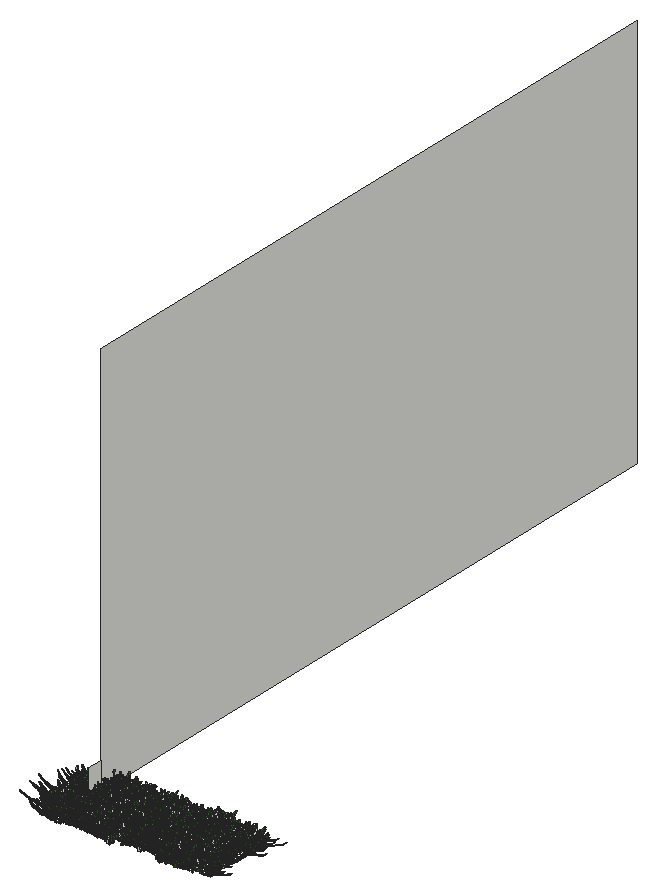
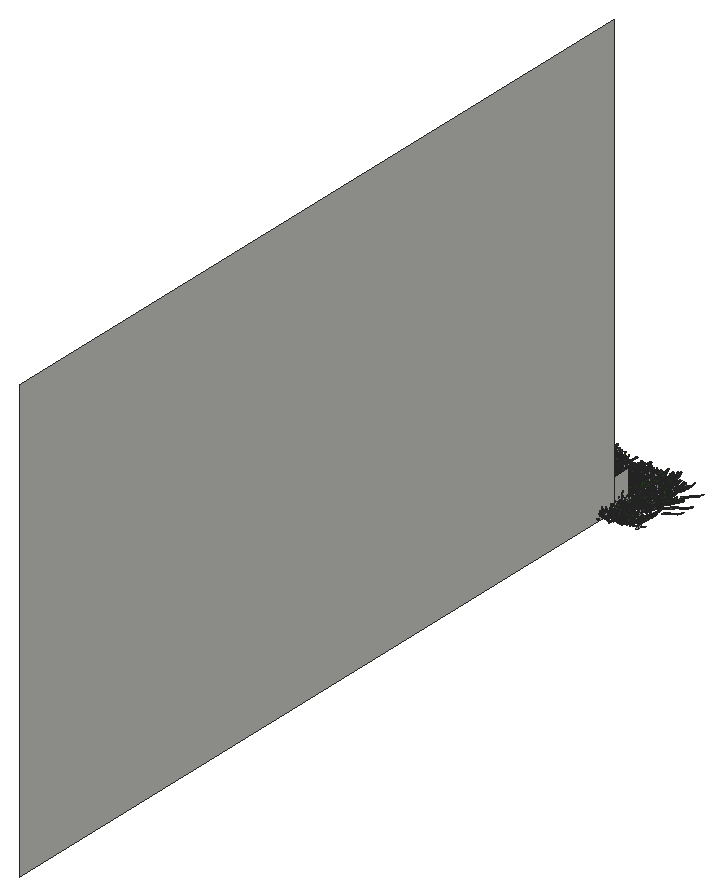
# SketchUp Ruby script. Lengths in inches.
U = 1.inch
M = Sketchup.active_model
def pt(a) = Geom::Point3d.new(a.map { |v| v * U })
def face(e, loops, mat)
  f = e.add_face(loops[0].map { |a| pt(a) })
  loops[1..].each { |l| e.add_face(l.map { |a| pt(a) }).erase! }
  f.material = f.back_material = mat if mat
  f
end
# faces: each face lists its corners as indices into pts; further lists are holes
def faces(e, pts, list, mat = nil) = list.each { |f| face(e, (f[0].is_a?(Array) ? f : [f]).map { |l| l.map { |i| pts[i] } }, mat) }
# xy, xz, yz: faces in a plane at the given z, y or x. An outline is a flat list of corners, or four numbers for a rectangle; further outlines are holes
def ring(l) = l.size == 4 ? [[l[0], l[1]], [l[2], l[1]], [l[2], l[3]], [l[0], l[3]]] : l.each_slice(2).to_a
def flat(e, list, mat, &to3) = list.each { |f| face(e, (f[0].is_a?(Array) ? f : [f]).map { |l| ring(l).map { |u, v| to3.(u, v) } }, mat) }
def xy(e, z, list, mat = nil) = flat(e, list, mat) { |x, y| [x, y, z] }
def xz(e, y, list, mat = nil) = flat(e, list, mat) { |x, z| [x, y, z] }
def yz(e, x, list, mat = nil) = flat(e, list, mat) { |y, z| [x, y, z] }
def lines(e, pts, list) = list.each { |a, b| e.add_line(pt(pts[a]), pt(pts[b])) }
# prism: a flat outline (further loops are holes) pulled along v
def prism(e, loops, v, mat = nil)
  f = face(e, loops, mat); d = Geom::Vector3d.new(v.map { |x| x * U })
  f.pushpull(f.normal.samedirection?(d) ? d.length : -d.length)
end
def box(e, o, s, mat = nil) = prism(e, [[o, [o[0] + s[0], o[1], o[2]], [o[0] + s[0], o[1] + s[1], o[2]], [o[0], o[1] + s[1], o[2]]]], [0, 0, s[2]], mat)
def at(x, y, z, deg = 0) = Geom::Transformation.translation(pt([x, y, z])) * Geom::Transformation.rotation(ORIGIN, Z_AXIS, deg.degrees)
def axes(o, x, y, z) = Geom::Transformation.new([*x, 0, *y, 0, *z, 0, *pt(o).to_a, 1])
def part(name) = M.definitions.add(name)
# library, detail: a bought-in or finely detailed component or shape, given as its bounding box
def library(name, o, s) = part(name).tap { |d| box(d.entities, o, s) }
def detail(e, o, s) = box(e.add_group.entities, o, s)
def put(e, d, t, mat = nil) = e.add_instance(d, t).tap { |i| i.material = mat if mat }
def group(e, t, mat = nil) = e.add_group.tap { |g| g.transformation = t; g.material = mat if mat }.entities
root = M.entities
M.materials.add("Material82").color = [68, 110, 58]
M.materials.add("Material83").color = [48, 90, 38]
M.materials.add("Material84").color = [68, 110, 48]
M.materials.add("Material85").color = [48, 90, 48]
M.materials.add("Material86").color = [58, 110, 58]
M.materials.add("Material87").color = [58, 90, 38]
M.materials.add("Material88").color = [68, 100, 58]
M.materials.add("Material89").color = [48, 100, 38]
c1 = part("grass00")
p = [[-0.6875,0.15,0],[-0.56,0.08,5.52],[-0.04,0.03,2.76],[0.48,-0.02,0],[0.35,-0.02,5.52],[-0.1,-0.14,5.52],
  [-0.12,0.65,8.37],[-0.42,0.65,8.37]]
faces(c1.entities,p,[[0,1,2,3],[3,2,4],[1,5,2],[5,4,2],[1,6,5],[4,5,6],[7,6,1]])
c2 = part("Group16\#1")
put(c2.entities,c1,axes([1.44,-0.61,-0.01],[0.05352,0.12609,0],[-0.10704,0.04543,0.07239],[0.06664,-0.02828,0.11628]),"Material85")
put(c2.entities,c1,axes([0.76,-0.15,-0.01],[0.04676,0.24062,0],[-0.23162,0.04501,0.06642],[0.0652,-0.01267,0.23595]),"Material82")
put(c2.entities,c1,axes([0.79,0.01,-0.01],[-0.00606,0.34651,0],[-0.34381,-0.00602,0.0432],[0.04319,0.00076,0.34386]))
put(c2.entities,c1,axes([1,0.23,-0.01],[-0.07192,0.31144,0],[-0.28722,-0.06632,0.1236],[0.12043,0.02781,0.29478]),"Material84")
put(c2.entities,c1,axes([1.66,0.77,-0.01],[-0.13828,0.29651,0],[-0.21551,-0.1005,0.22471],[0.20365,0.09498,0.23779]),"Material89")
put(c2.entities,c1,axes([0.6875,0.52,-0.01],[-0.18126,0.24051,0],[-0.22746,-0.17142,0.09788],[0.07817,0.05891,0.28481]),"Material84")
put(c2.entities,c1,axes([0.68,0.78,-0.01],[-0.215,0.18688,0],[-0.12385,-0.14248,0.21334],[0.13995,0.16101,0.18878]),"Material82")
put(c2.entities,c1,axes([0.56,1,-0.01],[-0.13756,0.07624,0],[-0.06159,-0.11112,0.0927],[0.04494,0.08108,0.12705]),"Material84")
put(c2.entities,c1,axes([0.2,0.64,-0.01],[-0.23729,0.07254,0],[-0.05711,-0.18681,0.153],[0.04473,0.14632,0.19535]),"Material89")
put(c2.entities,c1,axes([0.0625,0.72,-0.01],[-0.28874,0.02525,0],[-0.02179,-0.24916,0.14647],[0.01276,0.14591,0.25012]),"Material82")
put(c2.entities,c1,axes([-0.08,0.62,-0.01],[-0.34089,-0.04187,0],[0.03255,-0.26504,0.216],[-0.02633,0.21439,0.26703]),"Material89")
put(c2.entities,c1,axes([-0.34,0.98,-0.01],[-0.14314,-0.0493,0],[0.04397,-0.12769,0.06843],[-0.02228,0.0647,0.13505]),"Material89")
put(c2.entities,c1,axes([-0.87,1.45,-0.01],[-0.23488,-0.14114,0],[0.13761,-0.22901,0.06087],[-0.03135,0.05217,0.26717]))
put(c2.entities,c1,axes([-0.72,0.77,-0.01],[-0.14208,-0.13251,0],[0.07209,-0.0773,0.16301],[-0.11118,0.11922,0.1057]),"Material89")
put(c2.entities,c1,axes([-0.62,0.43,-0.01],[-0.14845,-0.21203,0],[0.18654,-0.13061,0.12304],[-0.10079,0.07057,0.22772]),"Material82")
put(c2.entities,c1,axes([-0.68,0.29,-0.01],[-0.13639,-0.32136,0],[0.31723,-0.13464,0.05579],[-0.05136,0.0218,0.34462]),"Material83")
put(c2.entities,c1,axes([-0.64,0.125,-0.01],[-0.0458,-0.23569,0],[0.22124,-0.043,0.08276],[-0.08124,0.01579,0.22538]),"Material86")
put(c2.entities,c1,axes([-1.6,-0.03,-0.01],[0.00576,-0.32897,0],[0.27526,0.00482,0.18018],[-0.18015,-0.00315,0.2753]),"Material84")
put(c2.entities,c1,axes([-1.36,-0.31,-0.01],[0.05718,-0.24765,0],[0.18172,0.04196,0.17267],[-0.16825,-0.03885,0.1865]),"Material89")
put(c2.entities,c1,axes([-1.54,-0.72,-0.01],[0.06537,-0.14017,0],[0.13555,0.06321,0.03939],[-0.0357,-0.01665,0.14956]))
put(c2.entities,c1,axes([-1.19,-0.9,-0.01],[0.09597,-0.12735,0],[0.11214,0.08451,0.07557],[-0.06035,-0.04548,0.14042]),"Material88")
put(c2.entities,c1,axes([-0.47,-0.54,-0.01],[0.11588,-0.10072,0],[0.0618,0.0711,0.12124],[-0.07953,-0.0915,0.0942]))
put(c2.entities,c1,axes([-0.47,-0.84,-0.01],[0.11927,-0.0661,0],[0.06603,0.11913,0.00646],[-0.00313,-0.00565,0.13621]),"Material84")
put(c2.entities,c1,axes([-0.38,-1.24,-0.01],[0.28037,-0.08571,0],[0.0618,0.20215,0.20315],[-0.05939,-0.19428,0.21139]),"Material88")
put(c2.entities,c1,axes([-0.06,-0.66,-0.01],[0.22719,-0.01987,0],[0.01247,0.14255,0.17758],[-0.01547,-0.17691,0.1431]),"Material87")
put(c2.entities,c1,axes([0.11,-0.89,-0.01],[0.14882,0.01828,0],[-0.01058,0.08611,0.12229],[0.01491,-0.12138,0.08676]),"Material85")
put(c2.entities,c1,axes([0.25,-0.72,-0.01],[0.20481,0.07053,0],[-0.06206,0.18022,0.10291],[0.03351,-0.0973,0.1906]),"Material85")
put(c2.entities,c1,axes([0.85,-1.42,-0.01],[0.16481,0.09904,0],[-0.09472,0.15762,0.05616],[0.02893,-0.04814,0.18389]),"Material84")
put(c2.entities,c1,axes([1.01,-1.09,-0.01],[0.21858,0.20385,0],[-0.17495,0.1876,0.15339],[0.10462,-0.11218,0.25652]),"Material89")
put(c2.entities,c1,axes([1.01,-0.71,-0.01],[0.08733,0.12473,0],[-0.06445,0.04512,0.13037],[0.1068,-0.07477,0.07867]),"Material85")
c3 = part("Group15\#1")
put(c3.entities,c2,at(0,0,0))
c4 = part("3darcstudiotree_grass00\#1")
put(c4.entities,c3,at(0,0,0))
yz(root,1830.75,[[1040.81,-29.74,1046.93,-18.36],[1046.93,-29.74,1318.18,131.1875]])
put(root,c4,axes([1829.06,1025.45,-29.74],[3.43874,0.27286,0],[-0.6732,1.31953,-0.0192],[-0.02432,0.04768,1.64321]))
put(root,c4,axes([1850.86,1025.03,-29.74],[-4.04807,0.23611,0],[-0.60438,-1.61163,-0.04443],[-0.03837,-0.10233,1.82802]))
put(root,c4,axes([1830.99,1025.28,-29.74],[1.27855,1.29921,0],[-4.02019,0.61532,-0.04732],[-0.19364,0.02964,1.41896]))
put(root,c4,axes([1876.93,1025.53,-29.74],[-1.72673,1.11938,0],[-3.66172,-0.8785,-0.02284],[-0.09991,-0.02397,1.64481]))
put(root,c4,axes([1840.07,1026.65,-29.74],[1.05791,1.29898,0],[-3.4169,0.4328,-0.04361],[-0.24845,0.03147,1.60948]))
put(root,c4,axes([1883.16,1027.24,-29.74],[2.97779,-1.31333,0],[2.93322,1.03437,-0.03435],[0.15944,0.05623,1.83666]))
put(root,c4,axes([1853.07,1027.35,-29.74],[1.68348,-1.42,0],[3.90393,0.71983,-0.01397],[0.0682,0.01258,1.74087]))
put(root,c4,axes([1834.37,1027.47,-29.74],[-2.53432,-1.16731,0],[3.13366,-1.05813,-0.03189],[0.12006,-0.04054,1.53238]))
put(root,c4,axes([1843.53,1027.46,-29.74],[-1.68076,1.66641,0],[-3.14491,-0.49334,-0.04072],[-0.22908,-0.03594,1.53595]))
put(root,c4,axes([1870.01,1027.81,-29.74],[-3.64575,-0.40954,0],[1.09452,-1.51542,-0.03955],[0.07063,-0.09779,1.95202]))
put(root,c4,axes([1860.55,1027.78,-29.74],[-4.50339,0.12702,0],[-0.32923,-1.8154,-0.06114],[-0.02191,-0.12082,1.73764]))
put(root,c4,axes([1875.2,1028.21,-29.74],[3.9368,0.32867,0],[-0.7645,1.42421,-0.03259],[-0.03941,0.07343,1.61556]))
put(root,c4,axes([1847.6875,1028.19,-29.74],[-1.97756,-1.20873,0],[2.87461,-0.73146,-0.04434],[0.19177,-0.0488,1.31982]))
put(root,c4,axes([1887.05,1027.84,-29.74],[-0.96856,1.32293,0],[-4.17213,-0.47507,-0.01983],[-0.0846,-0.00963,1.44555]))
put(root,c4,axes([1864.66,1028.02,-29.74],[-4.11343,-0.37841,0],[0.77008,-1.30194,-0.01564],[0.01915,-0.03238,1.3694]))
put(root,c4,axes([1839.86,1029.24,-29.74],[3.30112,0.44872,0],[-1.07202,1.22659,-0.01199],[-0.02088,0.02389,1.31812]))
put(root,c4,axes([1830.78,1029.07,-29.74],[2.54447,1.0037,0],[-2.66541,1.05092,-0.04694],[-0.19938,0.07861,1.69685]))
put(root,c4,axes([1844.18,1029.17,-29.74],[1.71949,1.25443,0],[-3.5766,0.76249,-0.00296],[-0.01327,0.00283,1.55057]))
put(root,c4,axes([1876.63,1028.93,-29.74],[-0.85979,1.68043,0],[-3.51636,-0.27982,-0.00527],[-0.03686,-0.00293,1.91768]))
put(root,c4,axes([1850.77,1030.125,-29.74],[2.98286,-1.36319,0],[2.94856,1.00345,-0.04774],[0.23651,0.08049,1.91023]))
put(root,c4,axes([1828.93,1029.47,-29.74],[-4.5512,0.12899,0],[-0.29843,-1.6376,-0.01837],[-0.00647,-0.03552,1.53349]))
put(root,c4,axes([1881.41,1030.28,-29.74],[2.31859,-1.24057,0],[3.7429,1.08799,-0.00987],[0.04342,0.01262,1.9048]))
put(root,c4,axes([1854.45,1029.86,-29.74],[3.00883,1.26771,0],[-3.0504,1.12602,-0.05678],[-0.17699,0.06533,1.337]))
put(root,c4,axes([1866.68,1030.28,-29.74],[2.02967,-1.41693,0],[3.62772,0.8082,-0.05349],[0.29346,0.06538,1.96798]))
put(root,c4,axes([1872.01,1030.18,-29.74],[-1.26608,-1.23533,0],[3.94424,-0.62872,-0.05241],[0.25484,-0.04062,1.67241]))
put(root,c4,axes([1860.23,1030.22,-29.74],[-2.51394,1.47726,0],[-3.35133,-0.88701,-0.03945],[-0.17377,-0.04599,1.6047]))
put(root,c4,axes([1831,1031.4375,-29.74],[1.0408,-1.70786,0],[3.59221,0.34047,-0.00397],[0.02558,0.00242,1.83602]))
put(root,c4,axes([1883.58,1031.08,-29.74],[1.31466,1.33352,0],[-4.27103,0.65487,-0.01993],[-0.10773,0.01652,1.99239]))
put(root,c4,axes([1878.18,1031.4,-29.74],[3.99583,0.96728,0],[-1.88023,1.20803,-0.0354],[-0.13352,0.08578,1.94218]))
put(root,c4,axes([1850.01,1031.29,-29.74],[1.07934,1.49635,0],[-4.41478,0.49528,-0.01266],[-0.0607,0.00681,1.71446]))
put(root,c4,axes([1838.61,1031.48,-29.74],[-3.99444,-0.7583,0],[1.47781,-1.21073,-0.01121],[0.03612,-0.02959,1.89718]))
put(root,c4,axes([1870.57,1031.38,-29.74],[0.15484,1.66312,0],[-4.06716,0.05889,-0.05084],[-0.28361,0.00411,1.70302]))
put(root,c4,axes([1855.93,1031.78,-29.74],[1.72171,1.1824,0],[-3.73214,0.84521,-0.0451],[-0.23455,0.05312,1.93445]))
put(root,c4,axes([1866.68,1032.42,-29.74],[0.19619,-1.71635,0],[3.31321,0.0589,-0.03915],[0.30696,0.00546,1.95085]))
put(root,c4,axes([1844.27,1032.2,-29.74],[-0.66988,1.5554,0],[-4.19746,-0.28116,-0.06003],[-0.34231,-0.02293,1.84592]))
put(root,c4,axes([1827.87,1032.45,-29.74],[-1.94069,1.13311,0],[-3.87728,-1.03282,-0.01862],[-0.08293,-0.02209,1.88514]))
put(root,c4,axes([1855.73,1033.21,-29.74],[1.1935,-1.34336,0],[4.3339,0.59885,-0.02001],[0.09738,0.01346,1.77455]))
put(root,c4,axes([1859.48,1032.45,-29.74],[-2.50228,1.03927,0],[-3.36492,-1.26006,-0.01749],[-0.0653,-0.02445,1.7911]))
put(root,c4,axes([1869.52,1033.83,-29.74],[3.2454,-0.59836,0],[1.90263,1.60498,-0.04906],[0.1129,0.09524,1.82977]))
put(root,c4,axes([1850.8,1034.125,-29.74],[3.36205,-0.0702,0],[0.18049,1.34442,-0.02933],[0.01197,0.08919,1.97542]))
put(root,c4,axes([1886.46,1033.98,-29.74],[-3.24576,-0.77305,0],[1.70346,-1.11239,-0.04514],[0.15554,-0.10157,1.64638]))
put(root,c4,axes([1859.23,1033.62,-29.74],[-2.83529,0.94791,0],[-2.49489,-1.16063,-0.0209],[-0.0692,-0.03219,1.48072]))
put(root,c4,axes([1866.07,1033.95,-29.74],[-4.36996,-0.43983,0],[0.81337,-1.25688,-0.00096],[0.00152,-0.00235,1.58162]))
put(root,c4,axes([1830.5,1034.09,-29.74],[2.0306,1.51402,0],[-3.86929,0.80712,-0.01033],[-0.04249,0.00886,1.52631]))
put(root,c4,axes([1839.74,1034.66,-29.74],[4.32541,0.68003,0],[-1.26335,1.24977,-0.02018],[-0.04043,0.04,1.38364]))
put(root,c4,axes([1876.86,1034.46,-29.74],[-1.11192,1.29739,0],[-3.39488,-0.45252,-0.04196],[-0.24016,-0.03201,1.62262]))
put(root,c4,axes([1844.39,1034.66,-29.74],[-3.14118,-0.50543,0],[1.51948,-1.46871,-0.03312],[0.08056,-0.07787,1.94116]))
put(root,c4,axes([1883.68,1034.5,-29.74],[-3.94382,0.34286,0],[-0.79478,-1.42188,-0.01188],[-0.01845,-0.03301,1.99665]))
put(root,c4,axes([1828.35,1034.6,-29.74],[-4.08544,0.78173,0],[-2.02978,-1.64985,-0.06144],[-0.10479,-0.08517,1.3618]))
put(root,c4,axes([1865.87,1035.39,-29.74],[0.47621,-1.80202,0],[3.38439,0.1391,-0.02929],[0.17813,0.00732,1.55926]))
put(root,c4,axes([1881.05,1035.93,-29.74],[4.51376,-0.38644,0],[0.93116,1.69158,-0.03342],[0.04124,0.07493,1.91382]))
put(root,c4,axes([1848.85,1036.43,-29.74],[2.93855,-0.93601,0],[2.3882,1.16609,-0.03491],[0.14245,0.06955,1.84986]))
put(root,c4,axes([1836.66,1036.26,-29.74],[3.70843,0.7821,0],[-1.67561,1.2357,-0.00407],[-0.01146,0.00845,1.59208]))
put(root,c4,axes([1858.79,1036.17,-29.74],[-3.51736,-0.62046,0],[1.43276,-1.26324,-0.00732],[0.0191,-0.01684,1.68082]))
put(root,c4,axes([1875.17,1036.67,-29.74],[1.17526,-1.64902,0],[4.03097,0.44682,-0.04021],[0.21409,0.02373,1.73573]))
put(root,c4,axes([1872.9,1036.78,-29.74],[3.33693,-0.09981,0],[0.31842,1.6558,-0.06006],[0.02203,0.11454,1.53056]))
put(root,c4,axes([1843.34,1036.95,-29.74],[1.17971,-1.62892,0],[3.63954,0.40996,-0.01145],[0.05532,0.00623,1.42532]))
put(root,c4,axes([1853.65,1036.61,-29.74],[-2.4369,-0.91248,0],[2.76412,-1.14811,-0.01822],[0.07791,-0.03236,1.86907]))
put(root,c4,axes([1831.56,1036.76,-29.74],[-4.28311,0.42951,0],[-0.86146,-1.33607,-0.01716],[-0.03026,-0.04692,1.87475]))
put(root,c4,axes([1833.83,1037.51,-29.74],[3.93391,0.38635,0],[-0.92741,1.4687,-0.04825],[-0.05916,0.09369,1.45973]))
put(root,c4,axes([1845.58,1037.91,-29.74],[1.5424,-1.39232,0],[4.02917,0.6942,-0.02716],[0.11079,0.01909,1.46706]))
put(root,c4,axes([1854.29,1037.73,-29.74],[-3.14575,-1.33265,0],[2.56413,-0.94137,-0.04944],[0.22162,-0.08136,1.60821]))
put(root,c4,axes([1871.02,1037.98,-29.74],[3.16271,-0.89527,0],[1.91794,1.05379,-0.02763],[0.08663,0.0476,1.3256]))
put(root,c4,axes([1836.38,1037.89,-29.74],[2.84603,0.80034,0],[-2.3016,1.27293,-0.03635],[-0.10022,0.05543,1.41103]))
put(root,c4,axes([1861.87,1037.97,-29.74],[2.37182,1.09167,0],[-3.5393,1.19596,-0.05975],[-0.18065,0.06104,1.3909]))
put(root,c4,axes([1865.67,1038.71,-29.74],[1.48234,-1.44208,0],[4.35208,0.69577,-0.03495],[0.16928,0.02706,1.83937]))
put(root,c4,axes([1827.48,1038,-29.74],[-3.86986,1.0079,0],[-2.20275,-1.31539,-0.01955],[-0.05283,-0.03155,1.46911]))
put(root,c4,axes([1881.31,1038.87,-29.74],[2.23867,-1.3669,0],[3.69886,0.94218,-0.0579],[0.27243,0.06939,1.84885]))
put(root,c4,axes([1877.36,1038.61,-29.74],[-1.90503,-1.23869,0],[3.27066,-0.78232,-0.01057],[0.0584,-0.01397,1.85267]))
put(root,c4,axes([1847.99,1038.94,-29.74],[-2.84152,0.97731,0],[-2.62045,-1.18497,-0.0546],[-0.22213,-0.10045,1.84968]))
put(root,c4,axes([1845.67,1039.74,-29.74],[-2.28475,-0.97473,0],[2.77585,-1.01196,-0.01026],[0.04604,-0.01678,1.73127]))
put(root,c4,axes([1875.03,1039.7,-29.74],[1.07114,1.64692,0],[-4.05863,0.41055,-0.04684],[-0.20509,0.02075,1.41954]))
put(root,c4,axes([1839.48,1039.79,-29.74],[0.72726,1.40914,0],[-3.71927,0.29854,-0.02796],[-0.18755,0.01505,1.94708]))
put(root,c4,axes([1855.85,1040.33,-29.74],[-2.0126,-1.62184,0],[4.11765,-0.79471,-0.06506],[0.29073,-0.05611,1.70958]))
put(root,c4,axes([1848.16,1039.74,-29.74],[-3.10197,1.07124,0],[-2.38472,-1.07399,-0.00238],[-0.01101,-0.00496,1.90825]))
put(root,c4,axes([1865.35,1039.99,-29.74],[-3.67787,-0.26396,0],[0.66039,-1.43112,-0.02729],[0.03307,-0.07167,1.8715]))
put(root,c4,axes([1872.48,1040.55,-29.74],[-0.88129,-1.68738,0],[3.67182,-0.29826,-0.02826],[0.15697,-0.01275,1.59374]))
put(root,c4,axes([1833.03,1040.8125,-29.74],[-1.15236,-1.67434,0],[3.65122,-0.39084,-0.0298],[0.14551,-0.01558,1.43464]))
put(root,c4,axes([1882.52,1040.57,-29.74],[0.85919,1.59494,0],[-3.67668,0.30804,-0.01067],[-0.0678,0.00568,1.82972]))
put(root,c4,axes([1859.2,1041.01,-29.74],[0.845,1.5364,0],[-3.22221,0.27563,-0.00976],[-0.06274,0.00537,1.62508]))
put(root,c4,axes([1883.6875,1042.06,-29.74],[3.21747,0.34612,0],[-1.00705,1.45598,-0.00322],[-0.00588,0.0085,1.99197]))
put(root,c4,axes([1855.42,1042.35,-29.74],[2.05313,-1.14667,0],[3.04328,0.84748,-0.00946],[0.04471,0.01245,1.61646]))
put(root,c4,axes([1876.25,1042.28,-29.74],[-2.06721,-1.47479,0],[2.97534,-0.64864,-0.04183],[0.21369,-0.04658,1.48723]))
put(root,c4,axes([1862.14,1042.34,-29.74],[3.55632,0.05998,0],[-0.17821,1.64336,-0.05798],[-0.01271,0.11725,1.60438]))
put(root,c4,axes([1886.46,1042,-29.74],[-3.26011,-0.21751,0],[0.57833,-1.34815,-0.02254],[0.02017,-0.04702,1.39425]))
put(root,c4,axes([1843.51,1043.2,-29.74],[3.71353,-0.51552,0],[1.56304,1.75115,-0.03514],[0.05159,0.0578,1.55988]))
put(root,c4,axes([1865.22,1043.27,-29.74],[1.06558,-1.7102,0],[3.88793,0.37676,-0.05295],[0.33853,0.03281,1.97565]))
put(root,c4,axes([1827.04,1043.27,-29.74],[3.5779,0.22372,0],[-0.65952,1.64048,-0.02805],[-0.02776,0.06904,1.99488]))
put(root,c4,axes([1837.97,1043.23,-29.74],[-0.99859,-1.42329,0],[3.17499,-0.34645,-0.0133],[0.07574,-0.00827,1.45899]))
put(root,c4,axes([1833.26,1042.7,-29.74],[-2.82382,0.83563,0],[-2.68315,-1.4102,-0.02868],[-0.0714,-0.03753,1.39]))
put(root,c4,axes([1872.16,1043.07,-29.74],[-4.01729,-0.17274,0],[0.40562,-1.46709,-0.05296],[0.03317,-0.11998,1.62079]))
put(root,c4,axes([1849.03,1043.13,-29.74],[-1.96777,1.0795,0],[-3.29786,-0.93497,-0.0015],[-0.00541,-0.00153,1.35234]))
put(root,c4,axes([1866.34,1044.2,-29.74],[3.84561,-0.02617,0],[0.07345,1.67847,-0.0287],[0.00308,0.07036,1.98369]))
put(root,c4,axes([1842.84,1044.41,-29.74],[1.96372,-1.5045,0],[4.10696,0.83372,-0.06088],[0.26019,0.05282,1.6642]))
put(root,c4,axes([1855.7,1044.37,-29.74],[3.54187,-0.26159,0],[0.80325,1.69151,-0.05648],[0.04449,0.09368,1.39957]))
put(root,c4,axes([1837.77,1044.66,-29.74],[1.82247,1.66574,0],[-4.14446,0.70523,-0.02206],[-0.09849,0.01676,1.64521]))
put(root,c4,axes([1861.64,1044.38,-29.74],[-3.99369,0.93834,0],[-2.11578,-1.40055,-0.00882],[-0.02078,-0.01375,1.42641]))
put(root,c4,axes([1875.53,1044.57,-29.74],[-3.34892,0.63546,0],[-1.79553,-1.4717,-0.05656],[-0.12201,-0.10001,1.54444]))
put(root,c4,axes([1871.73,1044.64,-29.74],[-2.29973,1.37871,0],[-3.78776,-0.98265,-0.04701],[-0.18775,-0.04871,1.62457]))
put(root,c4,axes([1885.91,1045.39,-29.74],[4.21864,0.55626,0],[-1.1609,1.36932,-0.01696],[-0.03551,0.04188,1.81122]))
put(root,c4,axes([1849.58,1044.99,-29.74],[-0.80631,1.56039,0],[-4.1673,-0.33492,-0.00834],[-0.04436,-0.00356,1.72954]))
put(root,c4,axes([1881.76,1045.37,-29.74],[-3.37719,0.09425,0],[-0.3007,-1.67585,-0.01026],[-0.00386,-0.0215,1.70108]))
put(root,c4,axes([1834.06,1045.54,-29.74],[-1.94441,1.40342,0],[-3.94861,-0.85085,-0.04785],[-0.22127,-0.04768,1.77706]))
put(root,c4,axes([1882.67,1046.53,-29.74],[3.52188,-1.04915,0],[2.07703,1.0844,-0.01203],[0.05383,0.0281,1.91781]))
put(root,c4,axes([1860.45,1046.875,-29.74],[1.01558,-1.39222,0],[4.1939,0.47581,-0.0144],[0.07646,0.00867,1.80693]))
put(root,c4,axes([1847.89,1046.35,-29.74],[0.28845,1.63387,0],[-3.6901,0.10132,-0.01352],[-0.07291,0.002,1.49862]))
put(root,c4,axes([1830.66,1047.07,-29.74],[1.87129,-1.65871,0],[3.35394,0.58849,-0.03607],[0.16948,0.02974,1.41495]))
put(root,c4,axes([1886.34,1047.05,-29.74],[3.01548,-1.43579,0],[2.66285,0.86981,-0.04892],[0.23141,0.07559,1.59182]))
put(root,c4,axes([1877.66,1046.41,-29.74],[-3.21998,0.77713,0],[-2.13854,-1.37813,-0.04749],[-0.1058,-0.06818,1.3106]))
put(root,c4,axes([1870.09,1047.21,-29.74],[4.18213,-0.23196,0],[0.63555,1.78214,-0.01318],[0.01066,0.02989,1.98636]))
put(root,c4,axes([1842.66,1047.34,-29.74],[4.18444,0.27637,0],[-0.72897,1.71663,-0.00046],[-0.00033,0.00077,1.40239]))
put(root,c4,axes([1855.15,1047.39,-29.74],[3.48402,0.19943,0],[-0.6366,1.72969,-0.0224],[-0.01372,0.03729,1.41716]))
put(root,c4,axes([1839.88,1047.47,-29.74],[2.76674,0.9412,0],[-2.67302,1.22208,-0.02494],[-0.08686,0.03971,1.63549]))
put(root,c4,axes([1866.78,1047.78,-29.74],[1.32588,-1.61709,0],[3.49004,0.44505,-0.02554],[0.12415,0.01583,1.40467]))
put(root,c4,axes([1827.83,1047.58,-29.74],[3.90165,0.71674,0],[-1.5443,1.30747,-0.0112],[-0.02712,0.02296,1.5714]))
put(root,c4,axes([1839.39,1048.63,-29.74],[2.92757,-1.05075,0],[2.58194,1.11883,-0.00947],[0.03015,0.01306,1.36019]))
put(root,c4,axes([1861.61,1048.73,-29.74],[2.43403,-1.47369,0],[3.95187,1.01516,-0.04483],[0.17665,0.04538,1.66248]))
put(root,c4,axes([1848.04,1048.72,-29.74],[-0.61871,-1.33799,0],[4.52735,-0.32561,-0.01194],[0.05418,-0.0039,1.59034]))
put(root,c4,axes([1872.79,1048.99,-29.74],[-2.58829,-1.32174,0],[3.13096,-0.95358,-0.00917],[0.03927,-0.01196,1.60374]))
put(root,c4,axes([1884.3,1048.77,-29.74],[0.77928,1.7442,0],[-4.29167,0.29822,-0.04576],[-0.22745,0.0158,1.64855]))
put(root,c4,axes([1854.67,1048.96,-29.74],[-0.96871,1.48497,0],[-4.54289,-0.46091,-0.03008],[-0.14643,-0.01486,1.76703]))
put(root,c4,axes([1825.5625,1049.47,-29.74],[2.90547,0.96842,0],[-2.50521,1.16898,-0.00305],[-0.01073,0.00501,1.58836]))
put(root,c4,axes([1843.49,1049.27,-29.74],[-3.42471,-0.0278,0],[0.09598,-1.83904,-0.05231],[0.00587,-0.11256,1.90792]))
put(root,c4,axes([1832.85,1049.57,-29.74],[-1.92512,-1.14787,0],[3.14134,-0.81939,-0.00554],[0.02611,-0.00681,1.59445]))
put(root,c4,axes([1875.2,1049.59,-29.74],[2.80131,1.49669,0],[-2.81369,0.81906,-0.03251],[-0.16371,0.04766,1.64081]))
put(root,c4,axes([1866.0625,1050.04,-29.74],[-2.36734,0.93793,0],[-2.35302,-0.92369,-0.04592],[-0.18701,-0.07341,1.42994]))
put(root,c4,axes([1849.99,1050.73,-29.74],[-4.54557,-0.49368,0],[1.16722,-1.67149,-0.00177],[0.00248,-0.00355,1.73275]))
put(root,c4,axes([1865.68,1051.27,-29.74],[2.58784,1.12355,0],[-2.76399,0.99014,-0.01914],[-0.07187,0.02574,1.41957]))
put(root,c4,axes([1880.66,1051.83,-29.74],[3.2252,-1.24507,0],[3.05222,1.22967,-0.00616],[0.02183,0.0088,1.65812]))
put(root,c4,axes([1839.09,1051.09,-29.74],[-3.2702,-0.26148,0],[0.88726,-1.72581,-0.02938],[0.02304,-0.04482,1.3208]))
put(root,c4,axes([1833.57,1051.72,-29.74],[3.46613,-0.34597,0],[1.04996,1.63602,-0.03471],[0.05136,0.08002,1.93398]))
put(root,c4,axes([1887,1051.19,-29.74],[-1.83571,1.27258,0],[-3.25848,-0.73105,-0.04597],[-0.18825,-0.04223,1.32398]))
put(root,c4,axes([1872.72,1051.87,-29.74],[3.30404,-0.44467,0],[1.11823,1.29225,-0.02189],[0.05068,0.05857,1.86062]))
put(root,c4,axes([1858.3,1051.79,-29.74],[3.79709,-0.21086,0],[0.51761,1.44966,-0.04526],[0.04066,0.11387,1.7925]))
put(root,c4,axes([1853.4,1051.42,-29.74],[-1.13728,1.56272,0],[-3.25789,-0.36875,-0.04255],[-0.28342,-0.03208,1.76068]))
put(root,c4,axes([1842.18,1052.16,-29.74],[3.34396,-0.78628,0],[2.01461,1.33256,-0.01626],[0.05098,0.03372,1.80561]))
put(root,c4,axes([1875.71,1051.57,-29.74],[-3.32221,0.63503,0],[-1.46009,-1.18802,-0.04774],[-0.13797,-0.11226,1.66266]))
put(root,c4,axes([1837.89,1052.89,-29.74],[1.37568,-1.20584,0],[3.91752,0.6951,-0.04402],[0.22671,0.04023,1.81837]))
put(root,c4,axes([1860.11,1052.8,-29.74],[3.59871,0.46514,0],[-1.32691,1.59666,-0.04711],[-0.07156,0.0861,1.55738]))
put(root,c4,axes([1847.88,1053,-29.74],[-2.0544,-1.27697,0],[2.98947,-0.74801,-0.00968],[0.05342,-0.01337,1.73508]))
put(root,c4,axes([1886.82,1053.42,-29.74],[3.62221,-0.68496,0],[1.51778,1.24833,-0.03326],[0.08982,0.07387,1.64345]))
put(root,c4,axes([1878.05,1052.98,-29.74],[-0.69326,1.7064,0],[-4.31448,-0.27262,-0.01053],[-0.04979,-0.00315,1.56894]))
put(root,c4,axes([1873.36,1053.3125,-29.74],[2.26243,1.54744,0],[-3.43917,0.78203,-0.02249],[-0.10645,0.02421,1.62577]))
